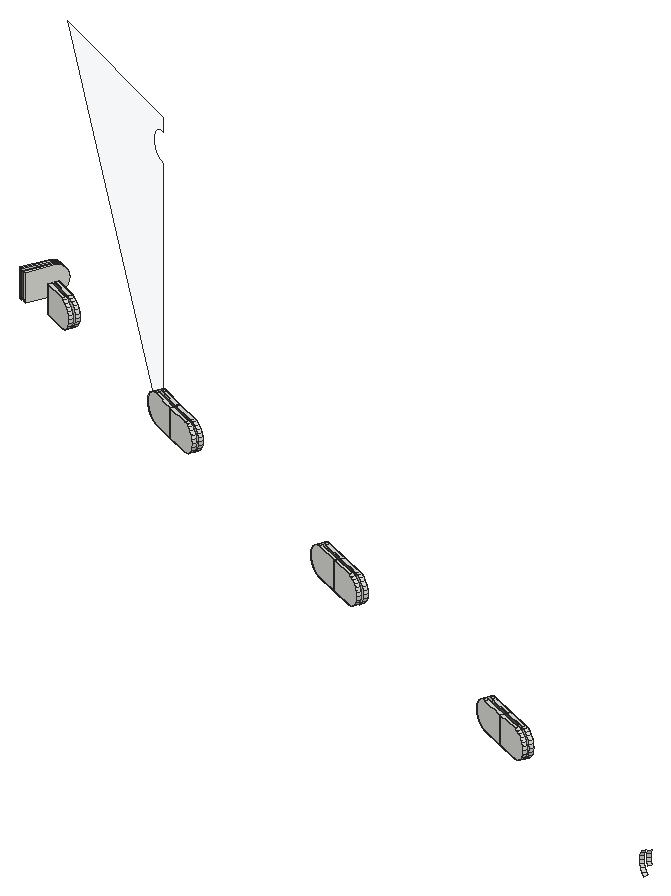
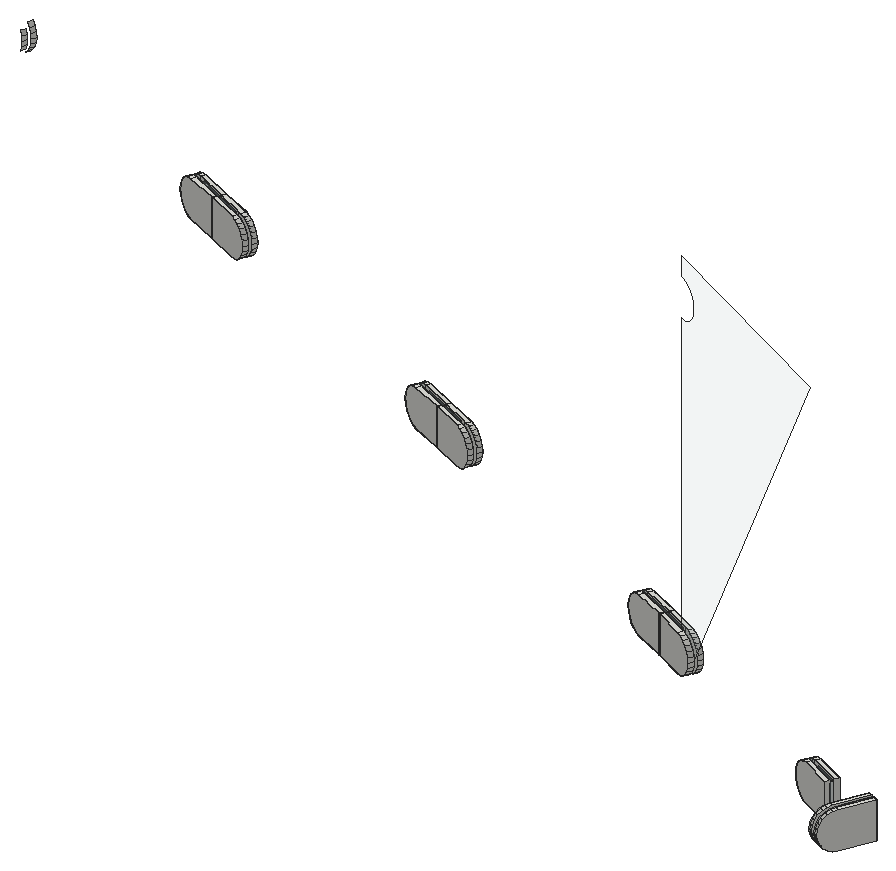
# SketchUp Ruby script. Lengths in inches.
U = 1.inch
M = Sketchup.active_model
def pt(a) = Geom::Point3d.new(a.map { |v| v * U })
def face(e, loops, mat)
  f = e.add_face(loops[0].map { |a| pt(a) })
  loops[1..].each { |l| e.add_face(l.map { |a| pt(a) }).erase! }
  f.material = f.back_material = mat if mat
  f
end
# faces: each face lists its corners as indices into pts; further lists are holes
def faces(e, pts, list, mat = nil) = list.each { |f| face(e, (f[0].is_a?(Array) ? f : [f]).map { |l| l.map { |i| pts[i] } }, mat) }
# xy, xz, yz: faces in a plane at the given z, y or x. An outline is a flat list of corners, or four numbers for a rectangle; further outlines are holes
def ring(l) = l.size == 4 ? [[l[0], l[1]], [l[2], l[1]], [l[2], l[3]], [l[0], l[3]]] : l.each_slice(2).to_a
def flat(e, list, mat, &to3) = list.each { |f| face(e, (f[0].is_a?(Array) ? f : [f]).map { |l| ring(l).map { |u, v| to3.(u, v) } }, mat) }
def xy(e, z, list, mat = nil) = flat(e, list, mat) { |x, y| [x, y, z] }
def xz(e, y, list, mat = nil) = flat(e, list, mat) { |x, z| [x, y, z] }
def yz(e, x, list, mat = nil) = flat(e, list, mat) { |y, z| [x, y, z] }
def lines(e, pts, list) = list.each { |a, b| e.add_line(pt(pts[a]), pt(pts[b])) }
# prism: a flat outline (further loops are holes) pulled along v
def prism(e, loops, v, mat = nil)
  f = face(e, loops, mat); d = Geom::Vector3d.new(v.map { |x| x * U })
  f.pushpull(f.normal.samedirection?(d) ? d.length : -d.length)
end
def box(e, o, s, mat = nil) = prism(e, [[o, [o[0] + s[0], o[1], o[2]], [o[0] + s[0], o[1] + s[1], o[2]], [o[0], o[1] + s[1], o[2]]]], [0, 0, s[2]], mat)
def at(x, y, z, deg = 0) = Geom::Transformation.translation(pt([x, y, z])) * Geom::Transformation.rotation(ORIGIN, Z_AXIS, deg.degrees)
def axes(o, x, y, z) = Geom::Transformation.new([*x, 0, *y, 0, *z, 0, *pt(o).to_a, 1])
def part(name) = M.definitions.add(name)
# library, detail: a bought-in or finely detailed component or shape, given as its bounding box
def library(name, o, s) = part(name).tap { |d| box(d.entities, o, s) }
def detail(e, o, s) = box(e.add_group.entities, o, s)
def put(e, d, t, mat = nil) = e.add_instance(d, t).tap { |i| i.material = mat if mat }
def group(e, t, mat = nil) = e.add_group.tap { |g| g.transformation = t; g.material = mat if mat }.entities
root = M.entities
M.materials.add("Glass_Safety_01").color = [204, 235, 244]
M.materials["Glass_Safety_01"].alpha = 0.1
xy(root,333,[[614.077,633.421,612.272,634.207,612.382,634.459,614.187,633.673],[614.266,633.854,612.461,634.64,612.571,634.892,614.376,634.106],[612.272,634.207,610.467,634.993,610.577,635.245,610.74,635.174,612.382,634.459],[612.461,634.64,610.819,635.355,610.656,635.426,610.766,635.678,612.571,634.892],[594.081,642.129,592.276,642.915,592.386,643.168,594.191,642.382],
  [594.27,642.5625,592.465,643.349,592.575,643.601,594.38,642.815],[592.276,642.915,590.471,643.701,590.581,643.954,590.746,643.883,592.386,643.168],[592.465,643.349,590.824,644.063,590.66,644.135,590.77,644.387,592.575,643.601],[574.269,650.758,572.464,651.544,572.574,651.797,574.379,651.011],[574.457,651.191,572.656,651.976,572.775,652.224,574.567,651.444],
  [572.452,651.55,570.677,652.401,570.796,652.65,570.999,652.552,572.571,651.798],[572.656,651.976,572.653,651.977,572.763,652.23,572.775,652.224],[572.653,651.977,571.084,652.73,570.881,652.827,571,653.076,572.763,652.23],[558.693,658.15,556.918,659.001,557.037,659.25,558.812,658.398],[558.897,658.576,557.122,659.427,557.241,659.675,559.016,658.824],
  [555.045,659.23,554.792,659.34,555.578,661.144,555.831,661.034],[554.612,659.418,554.359,659.528,555.145,661.333,555.398,661.223]])
xy(root,333.078,[[613.826,633.83,612.382,634.459,612.461,634.64,613.905,634.011],[612.382,634.459,610.938,635.088,611.017,635.269,612.461,634.64],[593.83,642.539,592.386,643.168,592.465,643.349,593.909,642.72],[592.386,643.168,590.942,643.797,591.021,643.977,592.465,643.349],[574.018,651.168,572.574,651.797,572.613,651.887,572.656,651.976,574.096,651.349],
  [572.571,651.798,571.151,652.48,571.236,652.657,572.653,651.977,572.613,651.887],[572.613,651.887,572.653,651.977,572.654,651.977,572.656,651.976],[558.457,658.568,557.037,659.25,557.122,659.427,558.542,658.746],[554.792,659.34,554.612,659.418,555.24,660.862,555.421,660.783]],"Glass_Safety_01")
xy(root,335.047,[[613.826,633.83,613.905,634.011,612.461,634.64,612.382,634.459],[612.382,634.459,612.461,634.64,611.017,635.269,610.938,635.088],[593.83,642.539,593.909,642.72,592.465,643.349,592.386,643.168],[592.386,643.168,592.465,643.349,591.021,643.977,590.942,643.797],[574.018,651.168,574.096,651.349,572.656,651.976,572.613,651.887,572.574,651.797],
  [572.571,651.798,572.613,651.887,572.653,651.977,571.236,652.657,571.151,652.48],[572.613,651.887,572.656,651.976,572.654,651.977,572.653,651.977],[558.457,658.568,558.542,658.746,557.122,659.427,557.037,659.25],[554.792,659.34,555.421,660.783,555.24,660.862,554.612,659.418]],"Glass_Safety_01")
xy(root,335.126,[[614.077,633.421,614.187,633.673,612.382,634.459,612.272,634.207],[614.266,633.854,614.376,634.106,612.571,634.892,612.461,634.64],[612.272,634.207,612.382,634.459,610.74,635.174,610.577,635.245,610.467,634.993],[612.461,634.64,612.571,634.892,610.766,635.678,610.656,635.426,610.819,635.355],[594.081,642.129,594.191,642.382,592.386,643.168,592.276,642.915],
  [594.27,642.5625,594.38,642.815,592.575,643.601,592.465,643.349],[592.276,642.915,592.386,643.168,590.746,643.883,590.581,643.954,590.471,643.701],[592.465,643.349,592.575,643.601,590.77,644.387,590.66,644.135,590.824,644.063],[574.269,650.758,574.379,651.011,572.574,651.797,572.464,651.544],[574.457,651.191,574.567,651.444,572.775,652.224,572.656,651.976],
  [572.452,651.55,572.571,651.798,570.999,652.552,570.796,652.65,570.677,652.401],[572.656,651.976,572.775,652.224,572.763,652.23,572.653,651.977],[572.653,651.977,572.763,652.23,571,653.076,570.881,652.827,571.084,652.73],[558.693,658.15,558.812,658.398,557.037,659.25,556.918,659.001],[558.897,658.576,559.016,658.824,557.241,659.675,557.122,659.427],
  [555.045,659.23,555.831,661.034,555.578,661.144,554.792,659.34],[554.612,659.418,555.398,661.223,555.145,661.333,554.359,659.528]])
p = [[614.077,633.421,335.126],[612.272,634.207,335.126],[612.272,634.207,333],[614.077,633.421,333],[614.329,633.311,333.036],[614.564,633.208,333.142],
  [614.766,633.12,333.311],[614.921,633.053,333.531],[615.018,633.011,333.787],[615.051,632.996,334.0625],[615.018,633.011,334.338],[614.921,633.053,334.594],
  [614.766,633.12,334.814],[614.564,633.208,334.983],[614.329,633.311,335.089],[614.187,633.673,335.126],[614.187,633.673,333],[614.439,633.563,333.036],
  [614.674,633.461,333.142],[614.876,633.373,333.311],[615.031,633.306,333.531],[615.128,633.263,333.787],[615.162,633.249,334.0625],[615.128,633.263,334.338],
  [615.031,633.306,334.594],[614.876,633.373,334.814],[614.674,633.461,334.983],[614.439,633.563,335.089],[614.266,633.854,333],[614.266,633.854,335.126],
  [614.518,633.744,335.089],[614.753,633.641,334.983],[614.955,633.554,334.814],[615.11,633.486,334.594],[615.207,633.444,334.338],[615.24,633.429,334.0625],
  [615.207,633.444,333.787],[615.11,633.486,333.531],[614.955,633.554,333.311],[614.753,633.641,333.142],[614.518,633.744,333.036],[614.628,633.997,333.036],
  [614.863,633.894,333.142],[612.382,634.459,335.126],[612.382,634.459,333],[612.382,634.459,333.078],[613.826,633.83,333.078],[613.826,633.83,335.047],
  [612.382,634.459,335.047],[612.571,634.892,335.126],[614.376,634.106,335.126],[614.628,633.997,335.089],[614.863,633.894,334.983],[615.065,633.806,334.814],
  [615.22,633.739,334.594],[615.317,633.696,334.338],[615.35,633.682,334.0625],[615.317,633.696,333.787],[615.22,633.739,333.531],[615.065,633.806,333.311],
  [614.376,634.106,333],[612.571,634.892,333],[612.461,634.64,333],[612.461,634.64,335.126],[612.461,634.64,335.047],[613.905,634.011,335.047],
  [613.905,634.011,333.078],[612.461,634.64,333.078],[610.467,634.993,335.126],[610.215,635.102,335.089],[609.98,635.205,334.983],[609.778,635.293,334.814],
  [609.623,635.36,334.594],[609.526,635.403,334.338],[609.493,635.417,334.0625],[609.526,635.403,333.787],[609.623,635.36,333.531],[609.778,635.293,333.311],
  [609.98,635.205,333.142],[610.215,635.102,333.036],[610.467,634.993,333],[610.74,635.174,333],[610.74,635.174,335.126],[610.938,635.088,335.047],
  [610.938,635.088,333.078],[610.819,635.355,335.126],[610.819,635.355,333],[611.017,635.269,333.078],[611.017,635.269,335.047],[610.766,635.678,335.126],
  [610.766,635.678,333],[610.514,635.788,333.036],[610.279,635.891,333.142],[610.077,635.979,333.311],[609.922,636.046,333.531],[609.825,636.088,333.787],
  [609.792,636.103,334.0625],[609.825,636.088,334.338],[609.922,636.046,334.594],[610.077,635.979,334.814],[610.279,635.891,334.983],[610.514,635.788,335.089],
  [610.325,635.355,333.036],[610.577,635.245,333],[610.09,635.458,333.142],[610.577,635.245,335.126],[609.888,635.545,333.311],[609.733,635.613,333.531],
  [609.636,635.655,333.787],[609.603,635.67,334.0625],[609.636,635.655,334.338],[609.733,635.613,334.594],[609.888,635.545,334.814],[610.09,635.458,334.983],
  [610.325,635.355,335.089],[610.656,635.426,333],[610.656,635.426,335.126],[610.404,635.536,335.089],[610.169,635.638,334.983],[609.967,635.726,334.814],
  [609.812,635.793,334.594],[609.715,635.836,334.338],[609.681,635.85,334.0625],[609.715,635.836,333.787],[609.812,635.793,333.531],[609.967,635.726,333.311],
  [610.169,635.638,333.142],[610.404,635.536,333.036],[594.081,642.129,335.126],[592.276,642.915,335.126],[592.276,642.915,333],[594.081,642.129,333],
  [594.333,642.02,333.036],[594.568,641.917,333.142],[594.77,641.829,333.311],[594.925,641.762,333.531],[595.022,641.719,333.787],[595.056,641.705,334.0625],
  [595.022,641.719,334.338],[594.925,641.762,334.594],[594.77,641.829,334.814],[594.568,641.917,334.983],[594.333,642.02,335.089],[594.443,642.272,333.036],
  [594.678,642.17,333.142],[594.191,642.382,333],[594.191,642.382,335.126],[594.88,642.082,333.311],[595.035,642.014,333.531],[595.132,641.972,333.787],
  [595.166,641.958,334.0625],[595.132,641.972,334.338],[595.035,642.014,334.594],[594.88,642.082,334.814],[594.678,642.17,334.983],[594.443,642.272,335.089],
  [594.27,642.5625,333],[594.27,642.5625,335.126],[594.522,642.453,335.089],[594.757,642.35,334.983],[594.959,642.262,334.814],[595.114,642.195,334.594],
  [595.211,642.153,334.338],[595.244,642.138,334.0625],[595.211,642.153,333.787],[595.114,642.195,333.531],[594.959,642.262,333.311],[594.757,642.35,333.142],
  [594.522,642.453,333.036],[592.386,643.168,335.126],[592.386,643.168,333],[592.386,643.168,333.078],[593.83,642.539,333.078],[593.83,642.539,335.047],
  [592.386,643.168,335.047],[592.575,643.601,335.126],[594.38,642.815,335.126],[594.632,642.705,335.089],[594.867,642.603,334.983],[595.069,642.515,334.814],
  [595.224,642.448,334.594],[595.321,642.405,334.338],[595.354,642.391,334.0625],[595.321,642.405,333.787],[595.224,642.448,333.531],[595.069,642.515,333.311],
  [594.867,642.603,333.142],[594.632,642.705,333.036],[594.38,642.815,333],[592.575,643.601,333],[592.465,643.349,333],[592.465,643.349,335.126],
  [592.465,643.349,335.047],[593.909,642.72,335.047],[593.909,642.72,333.078],[592.465,643.349,333.078],[590.471,643.701,335.126],[590.219,643.811,335.089],
  [589.984,643.914,334.983],[589.782,644.002,334.814],[589.627,644.069,334.594],[589.53,644.111,334.338],[589.497,644.126,334.0625],[589.53,644.111,333.787],
  [589.627,644.069,333.531],[589.782,644.002,333.311],[589.984,643.914,333.142],[590.219,643.811,333.036],[590.471,643.701,333],[590.746,643.883,333],
  [590.746,643.883,335.126],[590.942,643.797,335.047],[590.942,643.797,333.078],[590.824,644.063,335.126],[590.824,644.063,333],[591.021,643.977,333.078],
  [591.021,643.977,335.047],[590.77,644.387,335.126],[590.77,644.387,333],[590.518,644.497,333.036],[590.283,644.6,333.142],[590.081,644.6875,333.311],
  [589.926,644.755,333.531],[589.829,644.797,333.787],[589.796,644.812,334.0625],[589.829,644.797,334.338],[589.926,644.755,334.594],[590.081,644.6875,334.814],
  [590.283,644.6,334.983],[590.518,644.497,335.089],[590.329,644.064,333.036],[590.581,643.954,333],[590.094,644.166,333.142],[590.581,643.954,335.126],
  [589.892,644.254,333.311],[589.737,644.322,333.531],[589.64,644.364,333.787],[589.607,644.379,334.0625],[589.64,644.364,334.338],[589.737,644.322,334.594],
  [589.892,644.254,334.814],[590.094,644.166,334.983],[590.329,644.064,335.089],[590.66,644.135,333],[590.66,644.135,335.126],[590.408,644.244,335.089],
  [590.173,644.347,334.983],[589.971,644.435,334.814],[589.816,644.502,334.594],[589.719,644.545,334.338],[589.685,644.559,334.0625],[589.719,644.545,333.787],
  [589.816,644.502,333.531],[589.971,644.435,333.311],[590.173,644.347,333.142],[590.408,644.244,333.036],[574.269,650.758,335.126],[572.464,651.544,335.126],
  [572.464,651.544,333],[574.269,650.758,333],[574.521,650.648,333.036],[574.756,650.546,333.142],[574.958,650.458,333.311],[575.113,650.391,333.531],
  [575.21,650.348,333.787],[575.243,650.334,334.0625],[575.21,650.348,334.338],[575.113,650.391,334.594],[574.958,650.458,334.814],[574.756,650.546,334.983],
  [574.521,650.648,335.089],[574.631,650.901,333.036],[574.866,650.799,333.142],[574.379,651.011,333],[574.379,651.011,335.126],[575.068,650.711,333.311],
  [575.223,650.643,333.531],[575.32,650.601,333.787],[575.353,650.586,334.0625],[575.32,650.601,334.338],[575.223,650.643,334.594],[575.068,650.711,334.814],
  [574.866,650.799,334.983],[574.631,650.901,335.089],[574.457,651.191,335.126],[572.656,651.976,335.126],[572.656,651.976,335.047],[574.096,651.349,335.047],
  [574.096,651.349,333.078],[572.656,651.976,333.078],[572.656,651.976,333],[574.457,651.191,333],[574.71,651.082,333.036],[574.945,650.979,333.142],
  [575.147,650.891,333.311],[575.301,650.824,333.531],[575.399,650.781,333.787],[575.432,650.767,334.0625],[575.399,650.781,334.338],[575.301,650.824,334.594],
  [575.147,650.891,334.814],[574.945,650.979,334.983],[574.71,651.082,335.089],[572.574,651.797,335.126],[572.574,651.797,333],[572.574,651.797,333.078],
  [574.018,651.168,333.078],[574.018,651.168,335.047],[572.574,651.797,335.047],[572.763,652.23,335.126],[572.769,652.227,335.126],[572.775,652.224,335.126],
  [574.567,651.444,335.126],[574.82,651.334,335.089],[575.055,651.232,334.983],[575.257,651.144,334.814],[575.411,651.076,334.594],[575.509,651.034,334.338],
  [575.542,651.02,334.0625],[575.509,651.034,333.787],[575.411,651.076,333.531],[575.257,651.144,333.311],[575.055,651.232,333.142],[574.82,651.334,333.036],
  [574.567,651.444,333],[572.775,652.224,333],[572.769,652.227,333],[572.763,652.23,333],[572.452,651.55,335.126],[570.677,652.401,335.126],
  [570.429,652.52,335.089],[570.197,652.631,334.983],[569.999,652.726,334.814],[569.847,652.799,334.594],[569.751,652.845,334.338],[569.718,652.861,334.0625],
  [569.751,652.845,333.787],[569.847,652.799,333.531],[569.999,652.726,333.311],[570.197,652.631,333.142],[570.429,652.52,333.036],[570.677,652.401,333],
  [572.452,651.55,333],[572.571,651.798,333],[572.571,651.798,333.078],[572.571,651.798,335.047],[572.571,651.798,335.126],[570.999,652.552,333],
  [570.999,652.552,335.126],[571.151,652.48,335.047],[571.151,652.48,333.078],[572.653,651.977,333],[572.653,651.977,333.078],[571.236,652.657,333.078],
  [571.236,652.657,335.047],[572.653,651.977,335.047],[572.653,651.977,335.126],[571.084,652.73,335.126],[571.084,652.73,333],[572.654,651.977,333.078],
  [571,653.076,335.126],[571,653.076,333],[570.752,653.195,333.036],[570.521,653.306,333.142],[570.322,653.401,333.311],[570.17,653.474,333.531],
  [570.074,653.52,333.787],[570.042,653.535,334.0625],[570.074,653.52,334.338],[570.17,653.474,334.594],[570.322,653.401,334.814],[570.521,653.306,334.983],
  [570.752,653.195,335.089],[570.548,652.769,333.036],[570.796,652.65,333],[570.317,652.88,333.142],[570.796,652.65,335.126],[570.118,652.975,333.311],
  [569.966,653.048,333.531],[569.87,653.094,333.787],[569.837,653.11,334.0625],[569.87,653.094,334.338],[569.966,653.048,334.594],[570.118,652.975,334.814],
  [570.317,652.88,334.983],[570.548,652.769,335.089],[570.881,652.827,333],[570.633,652.946,333.036],[570.417,653.05,333.135],[569.924,653.286,334.049],
  [569.923,653.287,334.0625],[569.955,653.271,334.338],[570.051,653.225,334.594],[570.203,653.152,334.814],[570.402,653.057,334.983],[570.633,652.946,335.089],
  [570.881,652.827,335.126],[570.402,653.057,333.142],[558.693,658.15,335.126],[556.918,659.001,335.126],[556.918,659.001,333],[558.693,658.15,333],
  [558.941,658.031,333.036],[559.172,657.92,333.142],[559.37,657.825,333.311],[559.523,657.752,333.531],[559.618,657.706,333.787],[559.651,657.69,334.0625],
  [559.618,657.706,334.338],[559.523,657.752,334.594],[559.37,657.825,334.814],[559.172,657.92,334.983],[558.941,658.031,335.089],[558.812,658.398,335.126],
  [558.812,658.398,333],[559.06,658.279,333.036],[559.291,658.168,333.142],[559.489,658.073,333.311],[559.642,658,333.531],[559.738,657.954,333.787],
  [559.77,657.938,334.0625],[559.738,657.954,334.338],[559.642,658,334.594],[559.489,658.073,334.814],[559.291,658.168,334.983],[559.06,658.279,335.089],
  [558.897,658.576,333],[558.897,658.576,335.126],[559.145,658.457,335.089],[559.376,658.346,334.983],[559.575,658.251,334.814],[559.727,658.178,334.594],
  [559.823,658.132,334.338],[559.855,658.116,334.0625],[559.823,658.132,333.787],[559.727,658.178,333.531],[559.575,658.251,333.311],[559.376,658.346,333.142],
  [559.145,658.457,333.036],[559.264,658.705,333.036],[559.495,658.594,333.142],[557.037,659.25,335.126],[557.037,659.25,333],[557.037,659.25,333.078],
  [558.457,658.568,333.078],[558.457,658.568,335.047],[557.037,659.25,335.047],[557.241,659.675,335.126],[559.016,658.824,335.126],[559.264,658.705,335.089],
  [559.495,658.594,334.983],[559.694,658.499,334.814],[559.846,658.426,334.594],[559.942,658.38,334.338],[559.975,658.364,334.0625],[559.942,658.38,333.787],
  [559.846,658.426,333.531],[559.694,658.499,333.311],[559.016,658.824,333],[557.241,659.675,333],[557.122,659.427,333],[557.122,659.427,335.126],
  [557.122,659.427,335.047],[558.542,658.746,335.047],[558.542,658.746,333.078],[557.122,659.427,333.078],[554.792,659.34,333.078],[554.792,659.34,333],
  [555.045,659.23,333],[555.045,659.23,335.126],[554.792,659.34,335.126],[554.792,659.34,335.047],[555.831,661.034,335.126],[555.831,661.034,333],
  [555.941,661.287,333.036],[556.043,661.522,333.142],[556.131,661.723,333.311],[556.198,661.878,333.531],[556.241,661.976,333.787],[556.255,662.009,334.0625],
  [556.241,661.976,334.338],[556.198,661.878,334.594],[556.131,661.723,334.814],[556.043,661.522,334.983],[555.941,661.287,335.089],[555.578,661.144,335.126],
  [555.688,661.397,335.089],[555.79,661.632,334.983],[555.878,661.834,334.814],[555.946,661.988,334.594],[555.988,662.086,334.338],[556.002,662.119,334.0625],
  [555.988,662.086,333.787],[555.946,661.988,333.531],[555.878,661.834,333.311],[555.79,661.632,333.142],[555.688,661.397,333.036],[555.578,661.144,333],
  [555.421,660.783,333.078],[555.421,660.783,335.047],[554.612,659.418,333],[554.612,659.418,333.078],[554.612,659.418,335.047],[554.612,659.418,335.126],
  [554.359,659.528,335.126],[554.359,659.528,333],[555.398,661.223,335.126],[555.24,660.862,335.047],[555.24,660.862,333.078],[555.398,661.223,333],
  [555.507,661.475,333.036],[555.61,661.71,333.142],[555.698,661.912,333.311],[555.765,662.067,333.531],[555.808,662.164,333.787],[555.822,662.198,334.0625],
  [555.808,662.164,334.338],[555.765,662.067,334.594],[555.698,661.912,334.814],[555.61,661.71,334.983],[555.507,661.475,335.089],[555.145,661.333,335.126],
  [555.255,661.585,335.089],[555.357,661.82,334.983],[555.445,662.022,334.814],[555.512,662.177,334.594],[555.555,662.274,334.338],[555.569,662.308,334.0625],
  [555.555,662.274,333.787],[555.512,662.177,333.531],[555.445,662.022,333.311],[555.357,661.82,333.142],[555.255,661.585,333.036],[555.145,661.333,333],
  [629.524,626.994,333.311],[629.726,626.906,333.142],[629.616,626.653,333.142],[629.414,626.741,333.311],[572.613,651.887,333.078],[572.613,651.887,335.047],
  [572.654,651.977,335.047],[569.955,653.271,333.787],[570.051,653.225,333.531],[570.203,653.152,333.311],[629.369,627.061,333.531],[629.259,626.808,333.531],
  [629.272,627.103,333.787],[629.161,626.851,333.787],[629.447,627.242,333.531],[629.35,627.284,333.787],[629.46,627.537,333.787],[629.558,627.494,333.531],
  [629.238,627.118,334.0625],[629.128,626.865,334.0625],[629.317,627.298,334.0625],[629.427,627.551,334.0625],[571.084,652.73,351.283],[558.897,658.576,354.511],
  [571.084,652.73,354.511],[571.084,652.73,353.409],[570.881,652.827,353.409],[570.633,652.946,353.373],[570.402,653.057,353.267],[570.203,653.152,353.098],
  [570.051,653.225,352.877],[569.955,653.271,352.621],[569.923,653.287,352.346],[569.955,653.271,352.071],[570.051,653.225,351.815],[570.203,653.152,351.594],
  [570.402,653.057,351.425],[570.633,652.946,351.319],[570.881,652.827,351.283],[629.272,627.103,334.338],[629.161,626.851,334.338],[629.35,627.284,334.338],
  [629.46,627.537,334.338],[629.369,627.061,334.594],[629.259,626.808,334.594],[629.447,627.242,334.594],[629.558,627.494,334.594],[629.524,626.994,334.814],
  [629.414,626.741,334.814]]
faces(root,p,[[0,1,2,3,4,5,6,7,8,9,10,11,12,13,14],[17,18,5,4],[16,17,4,3],[39,40,41,42],[43,15,16,44,45,46,47,48],[49,50,51,52,53,54,55,56,57,58,59,42,41,60,61],[40,28,60,41],[62,28,29,63,64,65,66,67],
  [1,68,69,70,71,72,73,74,75,76,77,78,79,80,2],[44,45,48,43,1,2],[44,81,82,43,48,83,84,45],[63,85,86,62,67,87,88,64],[67,62,61,49,63,64],[89,49,61,90,91,92,93,94,95,96,97,98,99,100,101],[102,103,80,79],[104,102,79,78],
  [105,82,81,103,102,104,106,107,108,109,110,111,112,113,114],[115,86,85,116,117,118,119,120,121,122,123,124,125,126,127],[115,127,91,90],[127,126,92,91],[128,129,130,131,132,133,134,135,136,137,138,139,140,141,142],[143,144,133,132],[145,143,132,131],[169,146,145,170,171,172,173,174],
  [175,176,177,178,179,180,181,182,183,184,185,186,187,188,189],[167,168,187,186],[168,156,188,187],[190,156,157,191,192,193,194,195],[129,196,197,198,199,200,201,202,203,204,205,206,207,208,130],[170,171,174,169,129,130],[170,209,210,169,174,211,212,171],[191,213,214,190,195,215,216,192],
  [195,190,189,175,191,192],[217,175,189,218,219,220,221,222,223,224,225,226,227,228,229],[230,231,208,207],[232,230,207,206],[233,210,209,231,230,232,234,235,236,237,238,239,240,241,242],[243,214,213,244,245,246,247,248,249,250,251,252,253,254,255],[243,255,219,218],[255,254,220,219],
  [256,257,258,259,260,261,262,263,264,265,266,267,268,269,270],[271,272,261,260],[273,271,260,259],[284,285,286,287,288,289,290,291,292,293,294,295,296,297,298,299,300,301,302],[303,274,273,304,305,306,307,308],[309,310,311,312,313,314,315,316,317,318,319,320,321,322,323,324,325,326,327],[293,292,323,322],[292,291,324,323],
  [328,329,330,331,332,333,334,335,336,337,338,339,340,341,342],[343,344,345,346,328,342],[305,304,258,257,303,308],[343,347,348,346,345,349,350,344],[351,352,353,354,355,356,357,358],[285,356,355,352,351,290,289,286],[351,290,289,359,352],[351,352,355,356,309,327],
  [289,290,325,311,285,286],[360,309,327,361,362,363,364,365,366,367,368,369,370,371,372],[326,327,309,310,311,325],[373,374,341,340],[375,373,340,339],[376,348,347,374,373,375,377,378,379,380,381,382,383,384,385],[358,386,387,388,389,390,391,392,393,394,395,396,357],[386,387,362,361],
  [388,397,363,362,387],[398,399,400,401,402,403,404,405,406,407,408,409,410,411,412],[415,416,403,402],[414,415,402,401],[437,438,439,440],[441,413,414,442,443,444,445,446],[447,448,449,450,451,452,453,454,455,456,457,440,439,458,459],[438,426,458,439],
  [460,426,427,461,462,463,464,465],[443,442,400,399,441,446],[466,467,468,469,470,471],[472,469,468,473,474,475,476,477,478,479,480,481,482,483,484],[470,485,486,487,488,489,490,491,492,493,494,495,496,497,467,466,498,499,471],[500,501,502,503,504,505],[506,503,502,507,508,501,500,509,510,511,512,513,514,515,516,517,518,519,520],[460,465,462,461,447,459],
  [504,521,522,523,524,525,526,527,528,529,530,531,532,533,505],[497,496,474,473],[510,509,533,532],[496,495,475,474],[511,510,532,531],[534,535,536,537],[18,19,6,5],[38,39,42,59],
  [106,104,78,77],[126,125,93,92],[144,147,134,133],[166,167,186,185],[234,232,206,205],[254,253,221,220],[272,275,262,261],[294,293,322,321],
  [377,375,339,338],[397,543,364,363],[416,417,404,403],[436,437,440,457],[495,494,476,475],[512,511,531,530],[544,534,537,545],[19,20,7,6],
  [37,38,59,58],[107,106,77,76],[125,124,94,93],[147,148,135,134],[165,166,185,184],[235,234,205,204],[253,252,222,221],[275,276,263,262],
  [295,294,321,320],[378,377,338,337],[543,542,365,364],[417,418,405,404],[435,436,457,456],[494,493,477,476],[513,512,530,529],[546,544,545,547],
  [548,549,550,551],[20,21,8,7],[36,37,58,57],[108,107,76,75],[124,123,95,94],[148,149,136,135],[164,165,184,183],[236,235,204,203],
  [252,251,223,222],[276,277,264,263],[296,295,320,319],[379,378,337,336],[542,541,366,365],[418,419,406,405],[434,435,456,455],[493,492,478,477],
  [514,513,529,528],[552,546,547,553],[549,554,555,550],[21,22,9,8],[35,36,57,56],[109,108,75,74],[123,122,96,95],[149,150,137,136],
  [163,164,183,182],[237,236,203,202],[251,250,224,223],[277,278,265,264],[297,296,319,318],[380,379,336,335],[389,390,367,366,541],[419,420,407,406],
  [433,434,455,454],[492,491,479,478],[515,514,528,527],[573,552,553,574],[554,575,576,555],[22,23,10,9],[34,35,56,55],[110,109,74,73],
  [122,121,97,96],[150,151,138,137],[162,163,182,181],[238,237,202,201],[250,249,225,224],[278,279,266,265],[298,297,318,317],[381,380,335,334],
  [390,391,368,367],[420,421,408,407],[432,433,454,453],[491,490,480,479],[516,515,527,526],[577,573,574,578],[575,579,580,576],[23,24,11,10],
  [33,34,55,54],[111,110,73,72],[121,120,98,97],[151,152,139,138],[161,162,181,180],[239,238,201,200],[249,248,226,225],[279,280,267,266],
  [299,298,317,316],[382,381,334,333],[391,392,369,368],[421,422,409,408],[431,432,453,452],[490,489,481,480],[517,516,526,525],[581,577,578,582],
  [24,25,12,11],[32,33,54,53],[112,111,72,71],[120,119,99,98],[152,153,140,139],[160,161,180,179],[240,239,200,199],[248,247,227,226],
  [280,281,268,267],[300,299,316,315],[383,382,333,332],[392,393,370,369],[422,423,410,409],[430,431,452,451],[489,488,482,481],[518,517,525,524],
  [25,26,13,12],[31,32,53,52],[113,112,71,70],[119,118,100,99],[153,154,141,140],[159,160,179,178],[241,240,199,198],[247,246,228,227],
  [281,282,269,268],[301,300,315,314],[384,383,332,331],[393,394,371,370],[423,424,411,410],[429,430,451,450],[488,487,483,482],[519,518,524,523],
  [26,27,14,13],[30,31,52,51],[114,113,70,69],[118,117,101,100],[154,155,142,141],[158,159,178,177],[242,241,198,197],[246,245,229,228],
  [282,283,270,269],[302,301,314,313],[540,286,285,356,355],[385,384,331,330],[394,395,372,371],[424,425,412,411],[428,429,450,449],[487,486,484,483],
  [520,519,523,522],[27,15,0,14],[29,30,51,50],[105,114,69,68],[117,116,89,101],[155,146,128,142],[157,158,177,176],[233,242,197,196],
  [245,244,217,229],[283,274,256,270],[284,302,313,312],[376,385,330,329],[395,396,360,372],[425,413,398,412],[427,428,449,448],[486,485,472,484],
  [506,520,522,521]])
faces(root,p,[[15,16,17,18,19,20,21,22,23,24,25,26,27],[28,29,30,31,32,33,34,35,36,37,38,39,40],[146,145,143,144,147,148,149,150,151,152,153,154,155],[156,157,158,159,160,161,162,163,164,165,166,167,168],[274,273,271,272,275,276,277,278,279,280,281,282,283],[291,284,302,301,300,299,298,297,296,295,294,293,292],[413,414,415,416,417,418,419,420,421,422,423,424,425],[426,427,428,429,430,431,432,433,434,435,436,437,438],
  [46,45,48,47],[47,46,66,65],[67,66,65,64],[45,84,83,48],[64,48,45,67],[87,67,64,88],[84,83,88,87],[172,171,174,173],
  [173,172,194,193],[195,194,193,192],[171,212,211,174],[192,174,171,195],[215,195,192,216],[212,211,216,215],[306,305,308,307],[306,288,287,307],
  [287,286,289,288],[344,350,349,345],[344,538,539,345],[539,538,305,308],[538,539,355,352],[286,539,538,289],[354,355,352,353],[359,289,286,540,355,352],
  [350,349,354,353],[388,389,541,542,543,397],[444,443,446,445],[464,463,445,444],[465,464,463,462],[462,465,443,446],[502,501,466,471],[498,466,471,499],
  [501,508,507,502],[508,507,499,498],[556,357,396,395,394,393,392,391,390,389,557,558,559,560,561,562,563,564,565,566,567,568,569,570,571,572]],"Glass_Safety_01")
